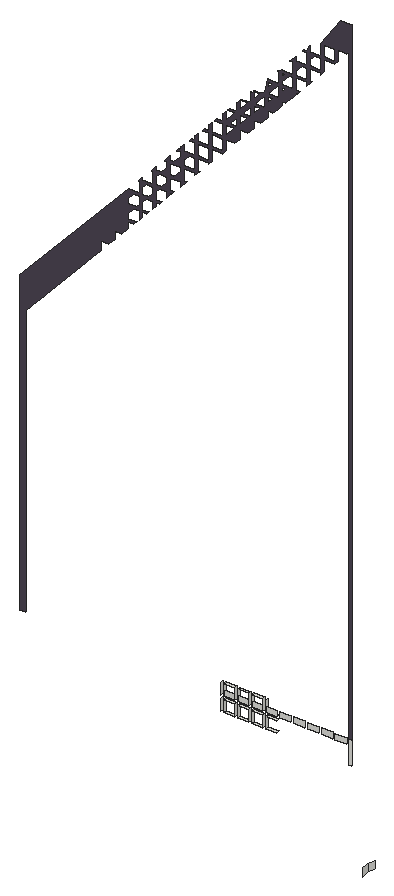
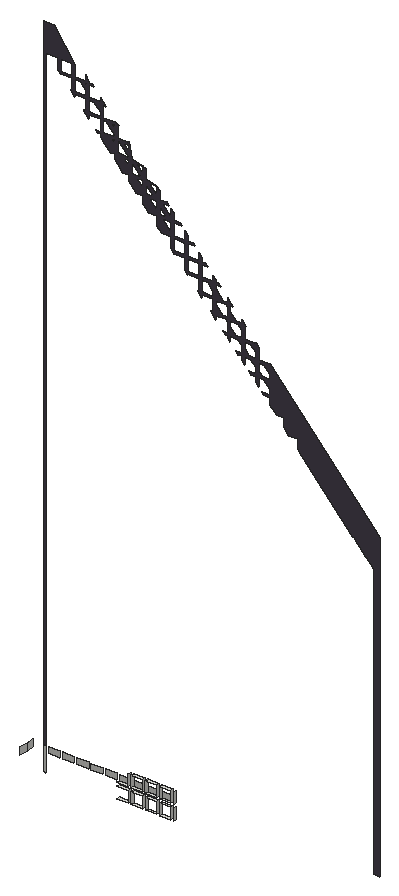
# SketchUp Ruby script. Lengths in inches.
U = 1.inch
M = Sketchup.active_model
def pt(a) = Geom::Point3d.new(a.map { |v| v * U })
def face(e, loops, mat)
  f = e.add_face(loops[0].map { |a| pt(a) })
  loops[1..].each { |l| e.add_face(l.map { |a| pt(a) }).erase! }
  f.material = f.back_material = mat if mat
  f
end
# faces: each face lists its corners as indices into pts; further lists are holes
def faces(e, pts, list, mat = nil) = list.each { |f| face(e, (f[0].is_a?(Array) ? f : [f]).map { |l| l.map { |i| pts[i] } }, mat) }
# xy, xz, yz: faces in a plane at the given z, y or x. An outline is a flat list of corners, or four numbers for a rectangle; further outlines are holes
def ring(l) = l.size == 4 ? [[l[0], l[1]], [l[2], l[1]], [l[2], l[3]], [l[0], l[3]]] : l.each_slice(2).to_a
def flat(e, list, mat, &to3) = list.each { |f| face(e, (f[0].is_a?(Array) ? f : [f]).map { |l| ring(l).map { |u, v| to3.(u, v) } }, mat) }
def xy(e, z, list, mat = nil) = flat(e, list, mat) { |x, y| [x, y, z] }
def xz(e, y, list, mat = nil) = flat(e, list, mat) { |x, z| [x, y, z] }
def yz(e, x, list, mat = nil) = flat(e, list, mat) { |y, z| [x, y, z] }
def lines(e, pts, list) = list.each { |a, b| e.add_line(pt(pts[a]), pt(pts[b])) }
# prism: a flat outline (further loops are holes) pulled along v
def prism(e, loops, v, mat = nil)
  f = face(e, loops, mat); d = Geom::Vector3d.new(v.map { |x| x * U })
  f.pushpull(f.normal.samedirection?(d) ? d.length : -d.length)
end
def box(e, o, s, mat = nil) = prism(e, [[o, [o[0] + s[0], o[1], o[2]], [o[0] + s[0], o[1] + s[1], o[2]], [o[0], o[1] + s[1], o[2]]]], [0, 0, s[2]], mat)
def at(x, y, z, deg = 0) = Geom::Transformation.translation(pt([x, y, z])) * Geom::Transformation.rotation(ORIGIN, Z_AXIS, deg.degrees)
def axes(o, x, y, z) = Geom::Transformation.new([*x, 0, *y, 0, *z, 0, *pt(o).to_a, 1])
def part(name) = M.definitions.add(name)
# library, detail: a bought-in or finely detailed component or shape, given as its bounding box
def library(name, o, s) = part(name).tap { |d| box(d.entities, o, s) }
def detail(e, o, s) = box(e.add_group.entities, o, s)
def put(e, d, t, mat = nil) = e.add_instance(d, t).tap { |i| i.material = mat if mat }
def group(e, t, mat = nil) = e.add_group.tap { |g| g.transformation = t; g.material = mat if mat }.entities
root = M.entities
M.materials.add("[Color M06]").color = [79, 71, 84]
xy(root,259.684,[[2246.43,480.141,2248.743,480.766],[2249.343,480.141,2251.655,480.766],[2252.255,480.141,2254.567,480.766],[2255.167,480.141,2257.479,480.766]])
xy(root,261.996,[[2246.43,480.141,2248.743,480.766],[2249.343,480.141,2251.655,480.766],[2252.255,480.141,2254.567,480.766],[2255.167,480.141,2257.479,480.766]])
xy(root,262.728,[[2246.459,480.141,2248.772,480.766],[2249.372,480.141,2251.684,480.766],[2252.284,480.141,2254.596,480.766],[2255.196,480.141,2257.508,480.766]])
xy(root,265.041,[[2246.459,480.141,2248.772,480.766],[2249.372,480.141,2251.684,480.766],[2252.284,480.141,2254.596,480.766]])
xz(root,480.141,[[2272.639,258.951,2273.215,263.889],[2246.459,262.728,2248.772,263.889],[2249.372,262.728,2251.684,263.889],[2252.284,262.728,2254.596,263.889],[2255.196,262.728,2257.508,263.889],
  [2258.108,262.728,2260.42,263.889],[2261.02,262.728,2263.332,263.889],[2263.932,262.728,2266.244,263.889],[2266.844,262.728,2269.156,263.889],[2269.756,262.728,2272.068,263.889]])
xz(root,480.141,[[[2203.903,263.889,2205.041,263.889,2205.041,320.238,2206.126,321.395,2206.657,321.962,2209.038,324.502,2209.038,324.774,2209.293,324.774,2217.774,333.822,2219.838,336.024,2220.686,336.929,2220.686,338.837,2222.474,338.837,2223.598,340.036,2223.598,341.649,2225.11,341.649,2226.51,343.143,2226.51,344.462,2227.746,344.462,2228.215,344.962,2226.51,344.962,2226.51,345.956,2227.746,347.274,2228.823,347.274,2228.823,345.61,2229.422,346.25,2229.422,347.274,2230.382,347.274,2230.851,347.774,2229.422,347.774,2229.422,349.0625,2230.382,350.087,2231.735,350.087,2231.735,348.717,2232.334,349.357,2232.334,350.087,2233.018,350.087,2233.487,350.587,2232.334,350.587,2232.334,352.169,2233.018,352.899,2234.647,352.899,2234.647,351.824,2235.246,352.464,2235.246,352.899,2235.654,352.899,2236.123,353.399,2235.246,353.399,2235.246,355.276,2235.654,355.712,2237.559,355.712,2237.559,354.931,2238.158,355.571,2238.158,355.712,2238.29,355.712,2238.759,356.212,2238.158,356.212,2238.158,358.524,2240.471,358.524,2240.471,358.038,2241.395,359.024,2241.07,359.024,2241.07,361.337,2243.383,361.337,2243.383,361.145,2244.031,361.837,2243.982,361.837,2243.982,364.149,2246.199,364.149,2246.894,364.891,2246.894,366.962,2248.835,366.962,2249.806,367.998,2249.806,369.774,2251.471,369.774,2251.94,370.274,2252.119,370.466,2252.718,371.105,2252.718,372.587,2254.107,372.587,2254.576,373.087,2255.031,373.573,2255.631,374.212,2255.631,375.399,2256.743,375.399,2257.153,375.837,2257.943,376.679,2258.543,377.319,2258.543,378.149,2259.321,378.149,2259.731,378.587,2260.855,379.786,2261.455,380.426,2261.455,380.899,2261.898,380.899,2262.308,381.337,2261.455,381.337,2261.455,383.649,2263.767,383.649,2263.767,382.893,2264.367,383.533,2264.367,383.649,2264.476,383.649,2264.565,383.746,2264.886,384.087,2264.367,384.087,2264.367,386.399,2266.679,386.399,2266.679,386,2267.463,386.837,2267.279,386.837,2267.279,389.149,2269.591,389.149,2269.591,389.107,2270.191,389.747,2270.191,391.899,2272.208,391.899,2272.639,392.359,2272.639,263.889,2273.215,263.889,2273.215,397.749,2270.965,397.749,2265.459,391.899,2266.679,391.899,2266.679,389.587,2264.367,389.587,2264.367,390.739,2263.767,390.102,2263.767,389.587,2263.282,389.587,2262.87,389.149,2263.767,389.149,2263.767,386.837,2261.455,386.837,2261.455,387.645,2260.855,387.008,2260.855,386.837,2260.693,386.837,2260.282,386.399,2260.855,386.399,2260.855,384.087,2258.543,384.087,2258.543,384.552,2257.693,383.649,2257.943,383.649,2257.943,381.337,2255.631,381.337,2255.631,381.458,2255.031,380.821,2255.031,378.587,2252.928,378.587,2252.119,377.727,2252.119,375.837,2250.339,375.837,2249.927,375.399,2251.471,375.399,2249.806,373.623,2249.806,375.271,2249.207,374.634,2249.207,373.087,2247.751,373.087,2247.28,372.587,2248.835,372.587,2246.894,370.516,2246.894,372.177,2246.295,371.54,2246.295,370.274,2245.103,370.274,2244.633,369.774,2246.295,369.774,2246.295,367.462,2243.982,367.462,2243.982,369.083,2243.383,368.447,2243.383,367.462,2242.456,367.462,2241.985,366.962,2243.383,366.962,2243.383,364.649,2241.07,364.649,2241.07,365.99,2240.471,365.353,2240.471,364.649,2239.808,364.649,2239.338,364.149,2240.471,364.149,2240.471,361.837,2238.158,361.837,2238.158,362.896,2237.559,362.259,2237.559,361.837,2237.161,361.837,2236.69,361.337,2237.559,361.337,2237.559,360.556,2236.123,359.024,2235.246,359.024,2235.246,359.803,2234.647,359.166,2234.647,359.024,2234.514,359.024,2234.043,358.524,2234.647,358.524,2234.647,357.449,2233.487,356.212,2232.334,356.212,2232.334,356.709,2231.396,355.712,2231.735,355.712,2231.735,353.399,2229.422,353.399,2229.422,353.615,2228.748,352.899,2228.823,352.899,2228.823,350.587,2226.571,350.587,2203.903,326.504],[2241.07,361.837,2243.383,364.149],[2243.982,364.649,2246.295,366.962],[2267.279,389.587,2269.591,391.899],[2264.367,386.837,2264.367,387.983,2265.464,389.149,2266.679,389.149,2266.679,386.837],[2238.158,359.024,2238.158,360.14,2239.284,361.337,2240.471,361.337,2240.471,359.024],[2229.422,350.587,2229.422,351.875,2230.382,352.899,2231.735,352.899,2231.735,351.53,2230.851,350.587],[2232.334,353.399,2232.334,354.982,2233.018,355.712,2234.647,355.712,2234.647,354.637,2233.487,353.399],[2226.51,347.774,2226.51,348.768,2227.746,350.087,2228.823,350.087,2228.823,348.423,2228.215,347.774],[2261.455,384.087,2261.455,384.89,2262.876,386.399,2263.767,386.399,2263.767,384.087],[2235.246,356.212,2235.246,358.089,2235.654,358.524,2237.559,358.524,2237.559,357.744,2236.123,356.212],[2258.543,381.337,2258.543,381.796,2260.287,383.649,2260.855,383.649,2260.855,381.337],[2255.631,378.587,2255.631,378.702,2257.698,380.899,2257.943,380.899,2257.943,378.587],[2252.933,375.837,2255.031,378.065,2255.031,375.837],[2246.894,367.704,2246.894,369.774,2248.835,369.774],[2250.345,373.087,2252.119,374.972,2252.119,373.087],[2249.806,370.811,2249.806,372.587,2251.471,372.587],[2247.697,370.274,2249.207,371.878,2249.207,370.274],[2252.718,373.918,2252.718,375.399,2254.107,375.399],[2252.718,376.668,2252.718,378.149,2254.107,378.149],[2255.631,376.962,2255.631,378.149,2256.743,378.149],[2255.631,379.712,2255.631,380.899,2256.743,380.899],[2258.543,380.069,2258.543,380.899,2259.321,380.899],[2258.543,382.819,2258.543,383.649,2259.321,383.649],[2237.108,359.024,2237.559,359.504,2237.559,359.024],[2261.455,385.926,2261.455,386.399,2261.898,386.399],[2234.46,356.212,2234.647,356.41,2234.647,356.212],[2238.158,361.196,2238.158,361.337,2238.29,361.337],[2264.367,389.033,2264.367,389.149,2264.476,389.149]]],"[Color M06]")
yz(root,2245.831,[[480.141,259.684,480.766,261.996]])
yz(root,2245.86,[[480.141,262.728,480.766,265.041]])
yz(root,2246.43,[[480.141,259.684,480.766,261.996]])
yz(root,2246.459,[[480.141,262.728,480.766,265.041]])
yz(root,2248.743,[[480.141,259.684,480.766,261.996]])
yz(root,2248.772,[[480.141,262.728,480.766,265.041]])
yz(root,2249.343,[[480.141,259.684,480.766,261.996]])
yz(root,2249.372,[[480.141,262.728,480.766,265.041]])
yz(root,2251.655,[[480.141,259.684,480.766,261.996]])
yz(root,2251.684,[[480.141,262.728,480.766,265.041]])
yz(root,2252.255,[[480.141,259.684,480.766,261.996]])
yz(root,2252.284,[[480.141,262.728,480.766,265.041]])
yz(root,2254.567,[[480.141,259.684,480.766,261.996]])
yz(root,2254.596,[[480.141,262.728,480.766,265.041]])
yz(root,2255.167,[[480.141,259.684,480.766,261.996]])
yz(root,2255.196,[[480.141,262.728,480.766,265.041]])
p = [[2288.517,463.841,250.875],[2288.3125,465.394,250.875],[2288.3125,465.394,252.375],[2288.517,463.841,252.375],[2288.517,466.947,250.875],[2288.517,466.947,252.375]]
faces(root,p,[[0,1,2,3],[1,4,5,2]])
